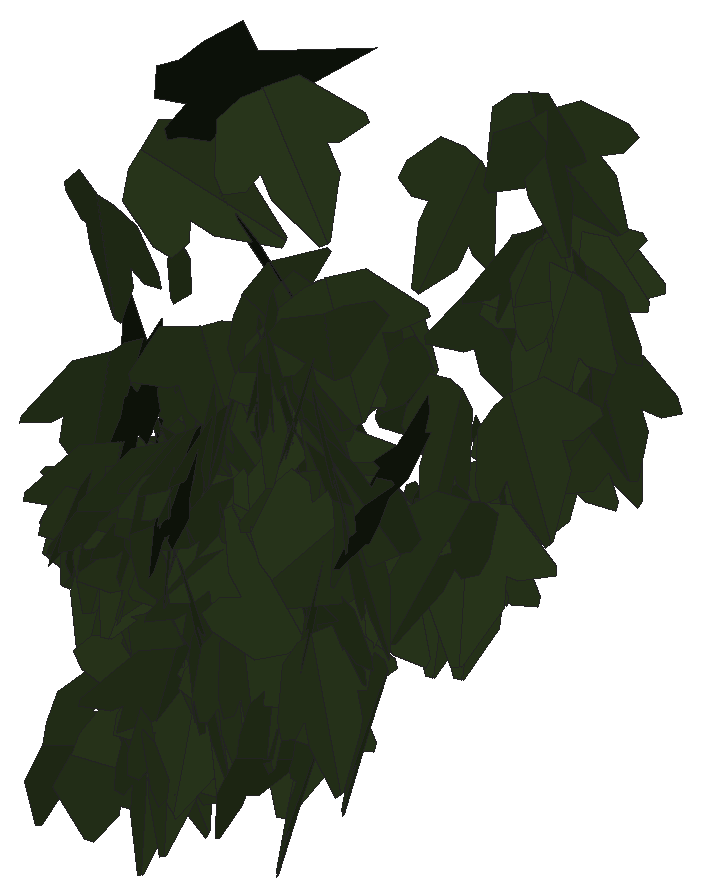
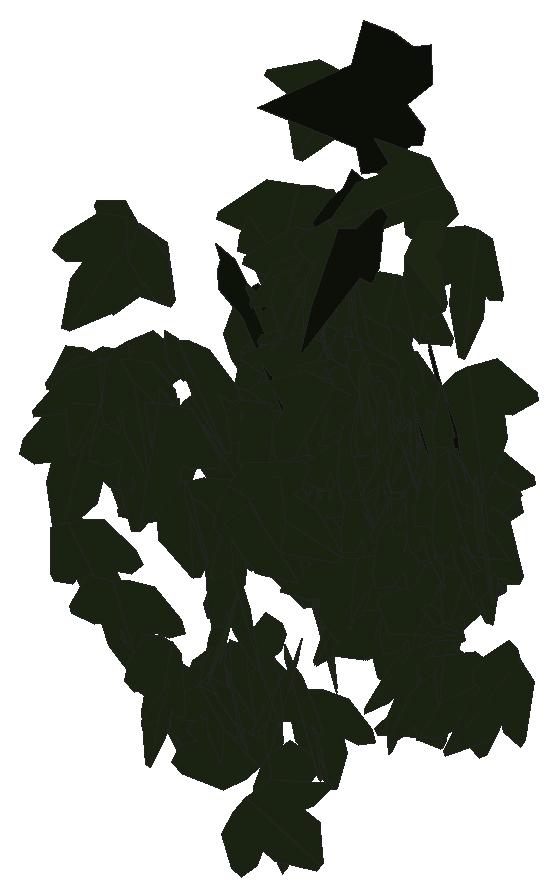
# SketchUp Ruby script. Lengths in inches.
U = 1.inch
M = Sketchup.active_model
def pt(a) = Geom::Point3d.new(a.map { |v| v * U })
def face(e, loops, mat)
  f = e.add_face(loops[0].map { |a| pt(a) })
  loops[1..].each { |l| e.add_face(l.map { |a| pt(a) }).erase! }
  f.material = f.back_material = mat if mat
  f
end
# faces: each face lists its corners as indices into pts; further lists are holes
def faces(e, pts, list, mat = nil) = list.each { |f| face(e, (f[0].is_a?(Array) ? f : [f]).map { |l| l.map { |i| pts[i] } }, mat) }
# xy, xz, yz: faces in a plane at the given z, y or x. An outline is a flat list of corners, or four numbers for a rectangle; further outlines are holes
def ring(l) = l.size == 4 ? [[l[0], l[1]], [l[2], l[1]], [l[2], l[3]], [l[0], l[3]]] : l.each_slice(2).to_a
def flat(e, list, mat, &to3) = list.each { |f| face(e, (f[0].is_a?(Array) ? f : [f]).map { |l| ring(l).map { |u, v| to3.(u, v) } }, mat) }
def xy(e, z, list, mat = nil) = flat(e, list, mat) { |x, y| [x, y, z] }
def xz(e, y, list, mat = nil) = flat(e, list, mat) { |x, z| [x, y, z] }
def yz(e, x, list, mat = nil) = flat(e, list, mat) { |y, z| [x, y, z] }
def lines(e, pts, list) = list.each { |a, b| e.add_line(pt(pts[a]), pt(pts[b])) }
# prism: a flat outline (further loops are holes) pulled along v
def prism(e, loops, v, mat = nil)
  f = face(e, loops, mat); d = Geom::Vector3d.new(v.map { |x| x * U })
  f.pushpull(f.normal.samedirection?(d) ? d.length : -d.length)
end
def box(e, o, s, mat = nil) = prism(e, [[o, [o[0] + s[0], o[1], o[2]], [o[0] + s[0], o[1] + s[1], o[2]], [o[0], o[1] + s[1], o[2]]]], [0, 0, s[2]], mat)
def at(x, y, z, deg = 0) = Geom::Transformation.translation(pt([x, y, z])) * Geom::Transformation.rotation(ORIGIN, Z_AXIS, deg.degrees)
def axes(o, x, y, z) = Geom::Transformation.new([*x, 0, *y, 0, *z, 0, *pt(o).to_a, 1])
def part(name) = M.definitions.add(name)
# library, detail: a bought-in or finely detailed component or shape, given as its bounding box
def library(name, o, s) = part(name).tap { |d| box(d.entities, o, s) }
def detail(e, o, s) = box(e.add_group.entities, o, s)
def put(e, d, t, mat = nil) = e.add_instance(d, t).tap { |i| i.material = mat if mat }
def group(e, t, mat = nil) = e.add_group.tap { |g| g.transformation = t; g.material = mat if mat }.entities
root = M.entities
M.materials.add("efeu1").color = [18, 25, 13]
M.materials.add("efeu2").color = [43, 57, 29]
c1 = part("ivyleaf_10")
p = [[0,0.5,-0.03],[-0.0625,2.02,-0.43],[-0.19,2.01,-0.46],[-0.54,1.05,-0.29],[-0.52,0.625,-0.18],[-0.83,0.76,-0.28],
  [-1.16,0.64,-0.33],[-1.15,0.33,-0.24],[-0.77,-0.39,0.02],[-0.3,-0.51,0.16],[0.04,-0.48,0.23],[-0.02,2.01,-0.4375],
  [-0.06,2.01,-0.43],[0.04,-0.49,0.23],[0.67,-0.49,0.14],[1.38,0.36,-0.2],[1.375,0.51,-0.24],[0.81,0.65,-0.19],
  [0.62,0.59,-0.15],[0.6,1.09,-0.28],[0.5,1.23,-0.31]]
faces(c1.entities,p,[[0,1,2,3,4,5,6,7,8,9,10],[11,12,0,13,14,15,16,17,18,19,20]],"efeu2")
c2 = part("ivyleaf_9")
p = [[1.54,2.16,1.25],[1.36,2.04,1.19],[-0.21,0.99,0.68],[-0.71,1.11,0.82],[-0.85,0.86,0.67],[-0.8,0.17,0.21],
  [-0.9,-0.01,0.1],[-0.67,-0.16,-0.02],[-0.08,-0.08,-0.05],[-0.03,-0.6,-0.4],[0.65,-0.88,-0.66],[0.83,-0.6,-0.49],
  [1.29,-0.42,-0.43],[1.8125,-0.07,-0.26],[1.21,0.44,0.15]]
faces(c2.entities,p,[[0,1,2,3,4,5,6,7,8,9,10,11,12,13,14]],"efeu1")
put(root,c1,axes([28.12,225.125,215.95],[0.05825,0.49632,0.01668],[0.0034,0.0164,-0.49972],[-0.49658,0.05833,-0.00146]))
put(root,c1,axes([27.125,225.24,217.54],[0.21426,-0.45021,-0.03747],[0.00768,-0.03784,0.49851],[-0.4517,-0.2142,-0.0093]))
put(root,c1,axes([25.93,225.23,217.6875],[-0.12932,-0.48294,0.00697],[0.0069,-0.00906,-0.49987],[0.48294,-0.12919,0.00901]))
put(root,c1,axes([28.5,225.28,215.75],[0.29908,-0.40033,0.01702],[0.00902,-0.0145,-0.49971],[0.40059,0.29921,-0.00145]))
put(root,c1,axes([27.54,225.18,218.59],[0.27499,-0.40942,-0.0822],[0.01469,0.10784,-0.48801],[0.41733,0.26598,0.07135]))
put(root,c1,axes([28.08,224.86,217.03],[0.1233,0.18011,-0.44984],[0.25447,0.37095,0.21827],[0.41236,-0.28277,-0.00018]))
put(root,c1,axes([27.02,225.17,218.3125],[-0.42821,-0.24018,-0.09461],[0.10627,0.00299,-0.48857],[0.23526,-0.43852,0.04849]))
put(root,c1,axes([28.16,225.16,218.86],[-0.32204,-0.37676,-0.06587],[0.03696,0.05505,-0.49558],[0.38069,-0.32407,-0.00761]))
put(root,c1,axes([26.05,225.125,219.13],[-0.46849,0.14781,0.0931],[-0.09382,0.01188,-0.49098],[-0.14735,-0.47751,0.0166]))
put(root,c2,axes([26.8,224.89,216.8],[0.03464,0.1079,0.48699],[-0.12703,0.47397,-0.09597],[-0.48235,-0.11708,0.06025]))
put(root,c1,axes([26.76,225.33,217.09],[-0.119,-0.48031,0.07171],[0.12339,-0.10131,-0.47383],[0.4697,-0.09507,0.14264]))
put(root,c1,axes([27.64,225.13,218.47],[-0.33724,0.36806,0.02832],[-0.02564,0.01491,-0.49912],[-0.36825,-0.3381,0.00881]))
put(root,c1,axes([27.85,225.29,218.46],[0.27947,0.39058,-0.13906],[-0.09054,-0.10616,-0.48014],[-0.4046,0.29355,0.01139]))
put(root,c1,axes([28.125,225.2,218.08],[-0.22806,0.43969,-0.0683],[0.04195,-0.05515,-0.49517],[-0.44298,-0.23159,-0.01173]))
put(root,c1,axes([27.91,225.36,216.62],[0.31103,-0.37641,0.10759],[0.09169,-0.06355,-0.48739],[0.3806,0.32292,0.02949]))
put(root,c1,axes([28.55,225.28,217.23],[-0.40343,0.01643,-0.29492],[-0.29456,0.01472,0.40376],[0.02195,0.49951,-0.0022]))
put(root,c1,axes([26.43,225.3,217.06],[-0.11906,-0.48498,0.02487],[0.00193,-0.02608,-0.49932],[0.48562,-0.1188,0.00808]))
put(root,c1,axes([27.88,225.21,218.34],[0.25192,-0.4065,-0.14593],[-0.05357,0.13822,-0.47752],[0.42856,0.25623,0.02609]))
put(root,c1,axes([26.49,225.32,215.28],[-0.17028,-0.46606,0.06161],[-0.0266,-0.05587,-0.49616],[0.46936,-0.17225,-0.00577]))
put(root,c1,axes([27.71,225.11,218.56],[-0.1222,0.47015,0.11843],[-0.13214,0.08522,-0.47463],[-0.46648,-0.1473,0.10342]))
put(root,c1,axes([27.76,225.16,218.8125],[-0.14168,0.47866,0.02846],[-0.015,0.02524,-0.49914],[-0.47927,-0.14229,0.00721]))
put(root,c1,axes([26.65,224.89,216.72],[-0.06019,0.13383,0.47798],[-0.23943,0.41394,-0.14605],[-0.4348,-0.24647,0.01426]))
put(root,c1,axes([26.57,225.43,216.95],[-0.1229,0.37931,-0.30169],[0.02459,-0.30596,-0.3947],[-0.48404,-0.11186,0.05655]))
put(root,c1,axes([26.74,225.3,216.76],[-0.3571,-0.34775,0.03934],[-0.02694,-0.02873,-0.49845],[0.34893,-0.35811,0.00178]))
put(root,c1,axes([27.6,225.21,220.47],[0.35829,0.26878,0.22223],[0.18468,0.12404,-0.44778],[-0.29584,0.40295,-0.01039]))
put(root,c1,axes([28.0625,225.27,217.39],[-0.36115,-0.33784,-0.07373],[0.08914,0.01206,-0.49184],[0.33411,-0.3684,0.05152]))
put(root,c1,axes([26.5625,225.45,216.93],[0.31062,-0.35608,0.16347],[0.12333,-0.10914,-0.4721],[0.37189,0.33361,0.02003]))
put(root,c1,axes([27.39,225.42,216.84],[-0.01137,0.02565,0.49921],[-0.43676,-0.24338,0.00255],[0.24313,-0.43601,0.02794]))
put(root,c1,axes([28.22,225.125,217.43],[0.17097,-0.03008,-0.4689],[-0.37792,0.28769,-0.15625],[0.27919,0.40784,0.07564]))
put(root,c1,axes([25.95,225.36,216.84],[-0.24085,-0.43612,0.0423],[0.01556,-0.05675,-0.49653],[0.43789,-0.23786,0.04091]))
put(root,c1,axes([25.875,225.37,216.18],[0.48967,-0.10108,-0.0011],[-0.00058,0.0026,-0.49999],[0.10109,0.48967,0.00243]))
put(root,c1,axes([26.08,225.39,216.51],[-0.35114,-0.2093,0.28792],[-0.24832,-0.14572,-0.40878],[0.25502,-0.43007,-0.00161]))
put(root,c1,axes([27.625,225.35,216.15],[0.16618,0.44132,0.16619],[-0.05611,-0.15645,0.47157],[0.46823,-0.17538,-0.00247]))
put(root,c1,axes([25.72,225.31,216.62],[0.17629,-0.45861,-0.09273],[-0.00716,0.09644,-0.49056],[0.46784,0.17429,0.02743]))
put(root,c1,axes([27.78,225.38,214.88],[0.28594,-0.40968,-0.02],[-0.01327,0.01513,-0.49959],[0.40995,0.28624,-0.00222]))
put(root,c1,axes([25.68,225,214.51],[-0.04172,-0.2221,-0.44602],[0.11959,0.43003,-0.22532],[0.48369,-0.12548,0.01724]))
put(root,c2,axes([28.82,225.0625,217.72],[-0.18971,0.39914,0.23388],[-0.09276,0.21483,-0.44186],[-0.45322,-0.21105,-0.00746]))
put(root,c1,axes([26.67,225.24,216.31],[-0.32781,0.37754,-0.00274],[0.00209,-0.00181,-0.49999],[-0.37754,-0.32781,-0.00039]))
put(root,c1,axes([27.77,225.26,218],[-0.46292,0.18739,-0.02426],[0.02187,-0.01063,-0.49941],[-0.18769,-0.46343,0.00164]))
put(root,c1,axes([26.78,225.39,217.25],[-0.14127,-0.47764,0.04364],[-0.00975,-0.04262,-0.49808],[0.47953,-0.14158,0.00272]))
put(root,c1,axes([26.82,225.32,217.59],[-0.4692,-0.00808,0.1726],[-0.17033,-0.06225,-0.46595],[0.02902,-0.49604,0.05566]))
put(root,c1,axes([27,225.32,217.77],[-0.40667,0.00526,-0.29085],[0.28787,-0.06464,-0.40367],[-0.04185,-0.49578,0.04955]))
put(root,c1,axes([25.95,225.38,216.57],[-0.01034,-0.49989,0.00116],[-0.00066,-0.00115,-0.5],[0.49989,-0.01034,-0.00064]))
put(root,c1,axes([26.98,225.39,217.57],[0.10156,-0.48955,-0.00522],[-0.00981,0.0033,-0.49989],[0.48948,0.10164,-0.00894]))
put(root,c1,axes([26.85,225.25,217.83],[0.35045,-0.26768,-0.23565],[-0.12903,0.21284,-0.43365],[0.33247,0.36475,0.0801]))
put(root,c1,axes([27.46,225.04,215],[-0.03118,-0.25266,-0.43034],[0.03237,0.42925,-0.25436],[0.49798,-0.04372,-0.01041]))
put(root,c1,axes([28.4,225.25,217.11],[-0.19935,0.45576,0.05042],[-0.02104,0.04583,-0.49745],[-0.45806,-0.20045,0.00091]))
put(root,c1,axes([26.89,225.3125,215.49],[-0.145,0.4777,-0.02787],[0.01017,-0.02604,-0.49922],[-0.47841,-0.14534,-0.00217]))
put(root,c1,axes([26.84,225.41,217.37],[-0.0417,-0.49792,-0.01846],[-0.00919,0.01929,-0.49954],[0.49817,-0.04132,-0.01076]))
put(root,c1,axes([27.05,225.4375,216.93],[-0.03916,-0.49816,0.01731],[0.00062,-0.01742,-0.4997],[0.49846,-0.03912,0.00198]))
put(root,c1,axes([26.33,225.38,216.82],[0.47306,-0.10586,-0.12251],[-0.10581,0.08422,-0.48136],[0.12255,0.48135,0.05728]))
put(root,c1,axes([26.01,225.36,216.57],[0.35891,0.33499,-0.09469],[-0.15711,0.0345,-0.47342],[-0.31065,0.36958,0.13003]))
put(root,c1,axes([25.97,225.17,214.38],[-0.14661,-0.15947,-0.45064],[0.37882,0.24872,-0.21127],[0.29154,-0.40337,0.04789]))
put(root,c1,axes([26.26,225.47,216.58],[0.02853,-0.4981,0.03297],[0.01283,-0.03228,-0.49879],[0.49902,0.0293,0.01094]))
put(root,c1,axes([28.14,225.25,219],[0.31383,0.36754,0.12816],[-0.00674,0.16972,-0.47026],[-0.38919,0.29344,0.11148]))
put(root,c1,axes([26.59,225.2,219.69],[0.17784,0.13699,0.44677],[0.3446,0.28443,-0.22439],[-0.31563,0.38773,0.00675]))
put(root,c1,axes([26.37,225.51,216.12],[-0.24995,-0.41693,0.11701],[-0.00319,-0.13333,-0.48188],[0.43303,-0.24164,0.06399]))
put(root,c1,axes([26.94,225.4375,216.26],[-0.09345,-0.49118,-0.00374],[0.0041,0.00303,-0.49997],[0.49117,-0.09347,0.00346]))
put(root,c1,axes([27.22,225.45,215.43],[0.49766,-0.01158,-0.0469],[-0.04668,0.00966,-0.49772],[0.01243,0.49977,0.00853]))
put(root,c1,axes([27.54,225.37,217.47],[-0.43199,0.10503,-0.2288],[0.22283,-0.052,-0.44457],[-0.11718,-0.48607,-0.00188]))
put(root,c1,axes([26.81,225.41,217.33],[-0.11424,-0.48555,-0.03451],[-0.00079,0.03563,-0.49873],[0.48677,-0.1139,-0.00891]))
put(root,c1,axes([25.8125,225.34,216.28],[-0.49743,0.00443,-0.05039],[0.05043,0.00459,-0.49743],[-0.00394,-0.49996,-0.00501]))
put(root,c2,axes([26.9375,225.08,220.48],[0.20631,0.10597,0.44295],[0.37448,0.23731,-0.23119],[-0.25923,0.42715,0.01855]))
put(root,c1,axes([26.89,225.4,217.44],[-0.05282,0.00739,-0.49715],[0.4941,-0.05501,-0.05331],[-0.05549,-0.49691,-0.00149]))
put(root,c1,axes([26.21,225.51,216.44],[0.38871,0.27567,-0.15138],[-0.11675,-0.09699,-0.47641],[-0.29202,0.40571,-0.01103]))
put(root,c1,axes([27.1,225.41,215.57],[0.078,0.49225,-0.04007],[-0.0017,-0.0403,-0.49837],[-0.49388,0.07788,-0.00461]))
put(root,c1,axes([26.2,225.51,214.49],[0.00412,0.46623,-0.18058],[-0.00969,-0.18048,-0.46619],[-0.49989,0.00734,0.00755]))
put(root,c1,axes([26.81,225.4,217.36],[-0.31818,-0.05812,-0.38129],[0.38491,-0.01622,-0.31872],[0.02468,-0.49635,0.05506]))
put(root,c1,axes([27.22,225.4,215.6875],[0.37928,-0.10093,-0.30977],[0.31423,-0.01225,0.38873],[-0.08606,-0.48955,0.05414]))
put(root,c1,axes([26.4,225.5,214.72],[0.06111,0.47655,-0.13845],[-0.01754,-0.13734,-0.48045],[-0.49594,0.06358,-0.00006]))
put(root,c1,axes([26.78,225.41,217.29],[0.11151,-0.47257,-0.11935],[-0.00212,0.12196,-0.48489],[0.4874,0.10864,0.0252]))
put(root,c1,axes([27.96,225.36,216.42],[-0.45491,0.15556,0.13733],[-0.13968,0.01515,-0.47985],[-0.15346,-0.47494,0.02967]))
put(root,c1,axes([27.12,225.38,216.56],[0.35916,0.34186,0.06428],[-0.00017,0.09257,-0.49136],[-0.34785,0.35293,0.06661]))
put(root,c1,axes([27.79,225.29,218.59],[0.29823,0.36308,0.17097],[0.01122,0.20539,-0.45573],[-0.40117,0.27566,0.11436]))
put(root,c1,axes([27.23,225.4,215.72],[-0.02207,0.49948,0.00554],[-0.00012,0.00554,-0.49997],[-0.49951,-0.02207,-0.00013]))
put(root,c1,axes([26.51,225.38,217.16],[-0.43617,0.24424,0.01022],[-0.00584,0.01049,-0.49986],[-0.24439,-0.43616,-0.0063]))
put(root,c1,axes([26.1,225.47,216.01],[0.38895,0.0459,0.31082],[0.30429,0.06819,-0.39084],[-0.07827,0.4932,0.02512]))
put(root,c1,axes([26.26,225.5,215.23],[0.19072,0.44065,0.13948],[-0.04775,-0.1313,0.48008],[0.45972,-0.19644,-0.008]))
put(root,c1,axes([26.53,225.46,215.55],[-0.41309,-0.2076,-0.19041],[0.20678,0.00604,-0.4552],[0.1913,-0.45482,0.08086]))
put(root,c2,axes([26.29,225.2,217.37],[-0.02031,0.09599,0.49028],[-0.13446,0.47153,-0.09789],[-0.48115,-0.13582,0.00666]))
put(root,c1,axes([27.77,225.35,217.46],[0.26143,0.36052,0.22732],[0.10611,0.20323,-0.44434],[-0.41279,0.28057,0.02976]))
put(root,c1,axes([26.59,225.52,215.01],[0.36742,0.33186,-0.0698],[-0.09048,-0.00326,-0.49173],[-0.32683,0.37397,0.05766]))
put(root,c1,axes([26.66,225.46,217.01],[-0.1581,0.47415,-0.01351],[0.00362,-0.01303,-0.49982],[-0.47433,-0.15814,0.00069]))
put(root,c1,axes([27.48,225.22,218.77],[0.04704,0.35621,0.34771],[-0.10715,0.34832,-0.34234],[-0.48611,-0.04231,0.10911]))
put(root,c1,axes([27.8,225.44,216.18],[-0.45902,0.12536,0.15356],[-0.14835,0.03968,-0.47583],[-0.13149,-0.4824,0.00076]))
put(root,c2,axes([27.14,225.43,219.28],[0.43784,-0.04948,-0.23632],[-0.23257,0.04503,-0.44032],[0.06485,0.4955,0.01642]))
put(root,c1,axes([26.49,225.38,218.97],[0.03483,0.08905,-0.49077],[-0.32512,0.37715,0.04536],[0.37826,0.31596,0.08418]))
put(root,c1,axes([26.35,225.51,214.6875],[-0.09064,0.47998,0.1068],[-0.00846,0.10707,-0.48833],[-0.49164,-0.09033,-0.01129]))
put(root,c1,axes([27.49,225.5625,217.18],[0.36687,0.25228,0.22751],[0.14169,0.1907,-0.43995],[-0.30876,0.38728,0.06843]))
put(root,c1,axes([27.99,225.72,216.88],[0.37838,0.32222,0.05481],[0.03979,0.0378,-0.49698],[-0.32441,0.38046,0.00296]))
put(root,c1,axes([26.85,225.91,215.66],[0.3503,0.35544,0.03077],[0.02346,0.02009,-0.49905],[-0.356,0.35108,-0.0026]))
put(root,c1,axes([28.56,226.17,216.87],[-0.12519,-0.41468,0.24973],[-0.02266,-0.25264,-0.43088],[0.48354,-0.1192,0.04446]))
put(root,c1,axes([27.74,226.17,216.03],[0.47693,0.06089,-0.13721],[-0.13508,-0.02528,-0.48074],[-0.06548,0.49563,-0.00766]))
put(root,c1,axes([26.74,226.67,214.58],[0.49619,0.06141,-0.00504],[-0.00471,-0.00299,-0.49997],[-0.06144,0.49621,-0.00239]))
put(root,c1,axes([28.22,226.76,216.41],[0.39187,0.31042,-0.00888],[-0.00776,-0.00451,-0.49992],[-0.31045,0.39195,0.00129]))
put(root,c1,axes([28.47,227.11,217.3],[0.09812,0.48065,0.09668],[-0.00594,0.09976,-0.48991],[-0.49024,0.09499,0.02529]))
put(root,c1,axes([26.79,227.59,217.21],[-0.1841,-0.15343,0.43882],[-0.32197,-0.29837,-0.2394],[0.33532,-0.37072,0.01106]))
put(root,c1,axes([26.3,227.49,215.37],[0.36116,-0.33857,-0.07021],[-0.04198,0.05785,-0.49487],[0.34322,0.36335,0.01336]))
put(root,c1,axes([27.42,227.55,216.8],[0.43093,-0.25357,0.00198],[0.01169,0.01596,-0.49961],[0.25331,0.43064,0.01969]))
put(root,c1,axes([28.21,227.57,219.6],[0.43711,-0.10467,0.21905],[0.23429,0.06368,-0.4371],[0.06361,0.48476,0.10472]))
put(root,c1,axes([26.59,227.74,217.2],[0.10757,0.42925,-0.23276],[-0.1566,-0.19543,-0.43277],[-0.4625,0.166,0.09239]))
put(root,c1,axes([28.35,227.71,218.0625],[0.49598,-0.00249,-0.06324],[-0.06326,-0.00434,-0.49596],[0.00192,0.49997,-0.00462]))
put(root,c1,axes([28.34,227.62,219.52],[-0.38038,-0.21526,-0.24285],[0.22322,0.09804,-0.43653],[0.23556,-0.44051,0.02151]))
put(root,c1,axes([27.36,227.79,218.6875],[0.45695,-0.16744,-0.11472],[-0.10994,0.03337,-0.48662],[0.17061,0.46995,-0.00632]))
put(root,c1,axes([28.04,227.84,218.38],[-0.04051,-0.49834,0.00416],[0.0081,-0.00484,-0.49991],[0.49829,-0.04044,0.00846]))
put(root,c1,axes([27.85,227.78,217.73],[-0.41276,-0.27831,-0.04657],[0.04171,0.02143,-0.4978],[0.27908,-0.41483,0.00552]))
put(root,c1,axes([26.66,228.02,215.45],[0.29921,-0.37229,0.14788],[0.14094,-0.07494,-0.47383],[0.37497,0.32524,0.0601]))
put(root,c1,axes([28.22,227.93,218.26],[0.4426,0.23227,-0.01243],[-0.01095,-0.00589,-0.49985],[-0.23234,0.44274,-0.00012]))
put(root,c1,axes([28.54,227.91,218.12],[-0.46589,0.18001,0.0233],[-0.0569,-0.08391,-0.48961],[-0.17236,-0.45886,0.09867]))
put(root,c1,axes([26.13,228.04,214.56],[0.04483,-0.49312,0.06942],[0.08978,-0.06055,-0.48813],[0.48983,0.05623,0.08312]))
put(root,c1,axes([26.77,227.98,215.52],[-0.19815,-0.45846,-0.0235],[0.00931,0.02158,-0.49945],[0.45896,-0.19837,-0.00001]))
put(root,c1,axes([26.06,227.9375,215.7],[-0.16195,0.4708,-0.0461],[0.02471,-0.04024,-0.49776],[-0.4724,-0.1635,-0.01024]))
put(root,c1,axes([28.32,228.02,218.26],[0.224,0.44112,-0.07235],[-0.02166,-0.07012,-0.49458],[-0.44649,0.22471,-0.0123]))
put(root,c1,axes([28.58,227.97,217.45],[-0.49475,-0.05376,-0.04834],[0.04972,-0.01028,-0.49742],[0.05249,-0.49699,0.01552]))
put(root,c1,axes([28.25,227.84,218.29],[0.13242,0.43828,0.20094],[0.06289,0.1909,-0.45782],[-0.47803,0.14652,-0.00457]))
put(root,c1,axes([26.96,228.09,215.28],[0.49794,-0.01162,0.04377],[0.0438,0.00096,-0.49808],[0.01149,0.49986,0.00197]))
put(root,c1,axes([26.55,228.06,214.79],[-0.19109,-0.3534,0.29765],[0.30856,0.14215,0.36686],[-0.34392,0.32389,0.16376]))
put(root,c1,axes([26.79,227.99,216.65],[-0.27373,0.14554,0.39229],[-0.38999,0.0811,-0.30222],[-0.1516,-0.47142,0.06912]))
put(root,c1,axes([26.7,228.08,216.33],[-0.34442,0.36238,-0.00776],[0.00778,-0.00331,-0.49993],[-0.36238,-0.34449,-0.00336]))
put(root,c1,axes([26.42,227.92,215.79],[0.12466,-0.01864,-0.48385],[-0.30001,0.3892,-0.09229],[0.38007,0.31333,0.08586]))
put(root,c1,axes([27.12,228.24,215.26],[0.49805,0.00666,0.04356],[0.0436,-0.00287,-0.49809],[-0.00638,0.49995,-0.00344]))
put(root,c1,axes([25.875,228.5625,214.5],[-0.24402,-0.28593,0.32969],[-0.01846,-0.37063,-0.33511],[0.43602,-0.17572,0.17032]))
put(root,c1,axes([26.89,228.29,215.5625],[0.05032,0.49363,-0.0616],[-0.00297,-0.06162,-0.49618],[-0.49745,0.0503,-0.00327]))
put(root,c1,axes([27.625,228.53,216.25],[0.4906,0.06114,-0.07466],[-0.07967,0.03831,-0.49212],[-0.05446,0.49477,0.04734]))
put(root,c1,axes([28.14,228.48,216.66],[0.428,-0.02817,-0.25695],[-0.24419,0.11895,-0.41979],[0.08478,0.48483,0.08806]))
put(root,c1,axes([27.03,228.66,215.78],[-0.44471,0.22068,0.05941],[-0.0626,0.00738,-0.49601],[-0.2198,-0.4486,0.02106]))
